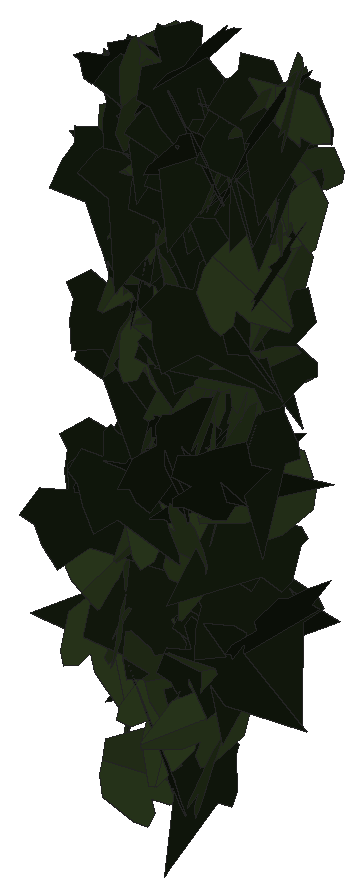
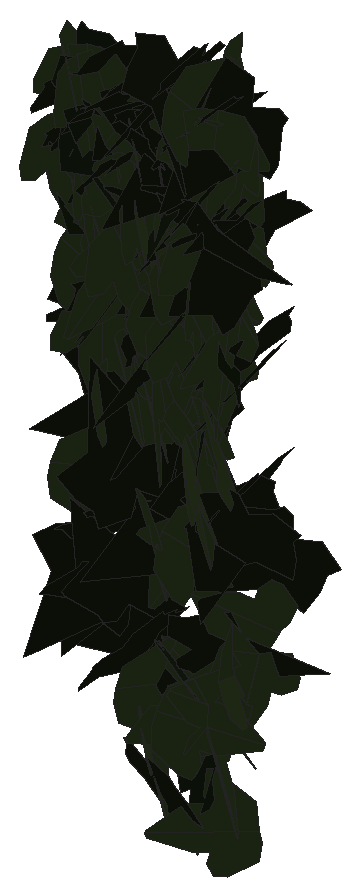
# SketchUp Ruby script. Lengths in inches.
U = 1.inch
M = Sketchup.active_model
def pt(a) = Geom::Point3d.new(a.map { |v| v * U })
def face(e, loops, mat)
  f = e.add_face(loops[0].map { |a| pt(a) })
  loops[1..].each { |l| e.add_face(l.map { |a| pt(a) }).erase! }
  f.material = f.back_material = mat if mat
  f
end
# faces: each face lists its corners as indices into pts; further lists are holes
def faces(e, pts, list, mat = nil) = list.each { |f| face(e, (f[0].is_a?(Array) ? f : [f]).map { |l| l.map { |i| pts[i] } }, mat) }
# xy, xz, yz: faces in a plane at the given z, y or x. An outline is a flat list of corners, or four numbers for a rectangle; further outlines are holes
def ring(l) = l.size == 4 ? [[l[0], l[1]], [l[2], l[1]], [l[2], l[3]], [l[0], l[3]]] : l.each_slice(2).to_a
def flat(e, list, mat, &to3) = list.each { |f| face(e, (f[0].is_a?(Array) ? f : [f]).map { |l| ring(l).map { |u, v| to3.(u, v) } }, mat) }
def xy(e, z, list, mat = nil) = flat(e, list, mat) { |x, y| [x, y, z] }
def xz(e, y, list, mat = nil) = flat(e, list, mat) { |x, z| [x, y, z] }
def yz(e, x, list, mat = nil) = flat(e, list, mat) { |y, z| [x, y, z] }
def lines(e, pts, list) = list.each { |a, b| e.add_line(pt(pts[a]), pt(pts[b])) }
# prism: a flat outline (further loops are holes) pulled along v
def prism(e, loops, v, mat = nil)
  f = face(e, loops, mat); d = Geom::Vector3d.new(v.map { |x| x * U })
  f.pushpull(f.normal.samedirection?(d) ? d.length : -d.length)
end
def box(e, o, s, mat = nil) = prism(e, [[o, [o[0] + s[0], o[1], o[2]], [o[0] + s[0], o[1] + s[1], o[2]], [o[0], o[1] + s[1], o[2]]]], [0, 0, s[2]], mat)
def at(x, y, z, deg = 0) = Geom::Transformation.translation(pt([x, y, z])) * Geom::Transformation.rotation(ORIGIN, Z_AXIS, deg.degrees)
def axes(o, x, y, z) = Geom::Transformation.new([*x, 0, *y, 0, *z, 0, *pt(o).to_a, 1])
def part(name) = M.definitions.add(name)
# library, detail: a bought-in or finely detailed component or shape, given as its bounding box
def library(name, o, s) = part(name).tap { |d| box(d.entities, o, s) }
def detail(e, o, s) = box(e.add_group.entities, o, s)
def put(e, d, t, mat = nil) = e.add_instance(d, t).tap { |i| i.material = mat if mat }
def group(e, t, mat = nil) = e.add_group.tap { |g| g.transformation = t; g.material = mat if mat }.entities
root = M.entities
M.materials.add("efeu1").color = [18, 25, 13]
M.materials.add("efeu2").color = [43, 57, 29]
c1 = part("ivyleaf_9")
p = [[1.54,2.16,1.25],[1.36,2.04,1.19],[-0.21,0.99,0.68],[-0.71,1.11,0.82],[-0.85,0.86,0.67],[-0.8,0.17,0.21],
  [-0.9,-0.01,0.1],[-0.67,-0.16,-0.02],[-0.08,-0.08,-0.05],[-0.03,-0.6,-0.4],[0.65,-0.88,-0.66],[0.83,-0.6,-0.49],
  [1.29,-0.42,-0.43],[1.8125,-0.07,-0.26],[1.21,0.44,0.15]]
faces(c1.entities,p,[[0,1,2,3,4,5,6,7,8,9,10,11,12,13,14]],"efeu1")
c2 = part("ivyleaf_10")
p = [[0,0.5,-0.03],[-0.0625,2.02,-0.43],[-0.19,2.01,-0.46],[-0.54,1.05,-0.29],[-0.52,0.625,-0.18],[-0.83,0.76,-0.28],
  [-1.16,0.64,-0.33],[-1.15,0.33,-0.24],[-0.77,-0.39,0.02],[-0.3,-0.51,0.16],[0.04,-0.48,0.23],[-0.02,2.01,-0.4375],
  [-0.06,2.01,-0.43],[0.04,-0.49,0.23],[0.67,-0.49,0.14],[1.38,0.36,-0.2],[1.375,0.51,-0.24],[0.81,0.65,-0.19],
  [0.62,0.59,-0.15],[0.6,1.09,-0.28],[0.5,1.23,-0.31]]
faces(c2.entities,p,[[0,1,2,3,4,5,6,7,8,9,10],[11,12,0,13,14,15,16,17,18,19,20]],"efeu2")
put(root,c1,axes([30.1875,223.73,218.27],[0.30823,0.1152,0.37646],[0.34662,0.14732,-0.32887],[-0.18669,0.46371,0.01096]))
put(root,c1,axes([30.05,223.875,220.49],[0.05189,-0.28466,-0.40777],[0.01949,0.41083,-0.28432],[0.49692,0.01361,0.05374]))
put(root,c2,axes([29.28,223.65,222.73],[0.01984,-0.0861,-0.49213],[-0.01626,0.49215,-0.08676],[0.49934,0.01944,0.01673]))
put(root,c1,axes([29.74,223.64,218.63],[-0.04067,0.07095,-0.49327],[-0.15542,0.46842,0.08019],[0.47349,0.15985,-0.01604]))
put(root,c1,axes([28.77,223.94,217.97],[0.27322,-0.33997,-0.24448],[-0.06771,0.25221,-0.42639],[0.41324,0.2661,0.09178]))
put(root,c1,axes([28.76,224.29,219.24],[0.07858,-0.48227,0.10603],[0.03475,-0.1017,-0.48831],[0.49256,0.08411,0.01754]))
put(root,c2,axes([30,224.4,215.17],[-0.10002,-0.01335,0.48971],[-0.07704,-0.49317,-0.02918],[0.4838,-0.08129,0.09659]))
put(root,c1,axes([29.83,224.33,222.33],[-0.24105,-0.43748,-0.0226],[0.01521,0.01743,-0.49946],[0.4378,-0.24148,0.0049]))
put(root,c1,axes([29.38,224.24,218.12],[0.19946,-0.19826,0.41341],[0.31844,-0.26446,-0.28047],[0.32987,0.37517,0.02077]))
put(root,c2,axes([29.8,224.47,219.83],[-0.07613,-0.08847,-0.48619],[-0.2503,-0.41725,0.11512],[-0.42609,0.26091,0.01924]))
put(root,c1,axes([29.32,224.45,217.93],[-0.04469,-0.06687,0.49349],[0.07031,-0.49136,-0.06021],[0.49301,0.06401,0.05332]))
put(root,c1,axes([29.86,223.93,222.43],[0.29147,0.04484,-0.40378],[-0.40614,0.04395,-0.2883],[0.00964,0.49604,0.06204]))
put(root,c1,axes([28.29,223.96,217.4],[0.01924,-0.08958,-0.49153],[0.23882,0.43371,-0.0697],[0.43885,-0.2321,0.05947]))
put(root,c2,axes([29.51,224.04,220.53],[-0.38484,0.31191,0.06791],[-0.07388,0.01645,-0.49424],[-0.31055,-0.39043,0.03343]))
put(root,c2,axes([29.62,224.43,219.1],[-0.1673,-0.31373,-0.35155],[-0.17157,-0.30688,0.35551],[-0.43883,0.23958,-0.00497]))
put(root,c2,axes([29.23,224.16,215.33],[-0.2636,-0.10284,0.41224],[0.41013,0.0651,0.27849],[-0.11095,0.48496,0.05004]))
put(root,c1,axes([28.61,224.24,219.85],[0.13988,-0.4487,-0.1706],[-0.039,0.16649,-0.46985],[0.47845,0.14475,0.01158]))
put(root,c1,axes([30.02,224.12,222.24],[0.03969,0.44035,-0.23348],[-0.01765,-0.23283,-0.44213],[-0.49811,0.04334,-0.00294]))
put(root,c1,axes([29.87,224.09,215.95],[0.06492,-0.00021,-0.49577],[0.37049,0.33227,0.04838],[0.32943,-0.37363,0.04329]))
put(root,c2,axes([30.46,223.94,220.87],[0.12331,0.35,0.3351],[0.09963,0.32008,-0.37097],[-0.4742,0.15826,0.0092]))
put(root,c1,axes([28.61,224.42,221.43],[-0.10626,-0.48093,-0.08611],[0.00554,0.08694,-0.49235],[0.48855,-0.10559,-0.01315]))
put(root,c2,axes([29.96,224.29,219.05],[0.23522,-0.43747,-0.05737],[-0.03723,0.0451,-0.49657],[0.43964,0.23788,-0.01135]))
put(root,c1,axes([29.8125,224.45,221.89],[-0.04801,-0.49268,-0.07041],[0.01432,0.06934,-0.49496],[0.49748,-0.04955,0.00746]))
put(root,c1,axes([29.07,224.57,222.47],[-0.09606,-0.47998,0.10192],[0.0028,-0.10439,-0.48897],[0.49068,-0.09337,0.02274]))
put(root,c1,axes([29.36,224.27,214.17],[0.16983,-0.32992,0.33513],[-0.1158,0.316,0.36977],[-0.45579,-0.20322,0.03092]))
put(root,c2,axes([29.8,224.1,217.06],[0.11381,-0.1009,-0.4763],[-0.36795,0.30251,-0.152],[0.31884,0.38511,-0.0054]))
put(root,c1,axes([28.9,224.59,221.3],[-0.15182,-0.4695,0.08071],[-0.01491,-0.07999,-0.49333],[0.47616,-0.15221,0.01029]))
put(root,c1,axes([30.49,224.4,218.87],[-0.31705,-0.08095,-0.37806],[0.36567,0.096,-0.32721],[0.12557,-0.48397,-0.00167]))
put(root,c2,axes([28.54,224.23,215.86],[0.2873,0.39943,0.08896],[0.04726,0.07558,-0.49199],[-0.40648,0.29111,0.00567]))
put(root,c2,axes([29.93,224.31,214.68],[0.20561,-0.44822,-0.08263],[-0.04335,0.071,-0.49303],[0.4537,0.20991,-0.00967]))
put(root,c1,axes([29.16,224.45,215.97],[-0.32167,-0.01003,0.38266],[-0.38267,-0.00433,-0.32179],[0.00977,-0.49988,-0.0049]))
put(root,c2,axes([29.6,224.44,219.01],[-0.31988,-0.21954,0.3154],[-0.2488,-0.19443,-0.38768],[0.29287,-0.40497,0.01515]))
put(root,c1,axes([28.78,224.52,220.21],[0.19828,-0.4454,0.11092],[0.03823,-0.10438,-0.48749],[0.45741,0.20179,-0.00734]))
put(root,c1,axes([30.43,224.54,222.28],[-0.0464,-0.49705,-0.028],[-0.00153,0.02826,-0.4992],[0.49784,-0.04624,-0.00414]))
put(root,c2,axes([29.15,224.35,218.8],[0.39495,-0.28137,-0.12183],[-0.09512,0.07644,-0.48488],[0.29149,0.40619,0.00685]))
put(root,c2,axes([28.98,224.54,220.58],[0.16357,0.32776,-0.34032],[-0.18287,-0.28816,-0.36541],[-0.43567,0.24401,0.0256]))
put(root,c2,axes([30.03,224.37,221.95],[0.22572,-0.4388,-0.08062],[-0.04065,0.06975,-0.49344],[0.44429,0.22932,-0.00419]))
put(root,c2,axes([28.47,224.52,220.23],[0.18963,-0.13955,-0.4411],[0.35215,-0.26564,0.23543],[-0.30006,-0.39995,-0.00246]))
put(root,c2,axes([28.91,224.24,219.64],[0.07968,-0.44012,-0.22349],[0.00451,0.22702,-0.44547],[0.49359,0.06898,0.04014]))
put(root,c2,axes([30.54,224.35,219.59],[-0.33784,-0.36837,-0.01319],[0.00837,0.01021,-0.49983],[0.36851,-0.33794,-0.00073]))
put(root,c1,axes([29.77,224.37,219.52],[-0.20294,-0.40635,0.20905],[0.12789,0.16909,0.45283],[-0.4387,0.23726,0.03531]))
put(root,c1,axes([28.9,224.14,217.875],[0.27649,0.40731,-0.08747],[-0.04935,-0.07222,-0.49229],[-0.41366,0.28086,0.00027]))
put(root,c1,axes([29.4375,224.11,222.98],[0.29733,-0.13893,-0.37722],[-0.17794,0.37524,-0.27845],[0.36046,0.29983,0.1737]))
put(root,c2,axes([29.13,224.67,222.81],[-0.00769,-0.35915,0.34778],[0.02542,-0.34765,-0.35846],[0.49929,0.01217,0.02361]))
put(root,c1,axes([30.7,224.66,219.77],[-0.35779,-0.08307,0.33925],[-0.30073,-0.17371,-0.3597],[0.17762,-0.46144,0.07434]))
put(root,c2,axes([29.17,224.27,219.6],[0.16895,0.45543,0.11848],[0.04351,0.11023,-0.48575],[-0.46857,0.17445,-0.00238]))
put(root,c2,axes([29.32,224.44,215.08],[0.38699,0.3021,-0.09474],[-0.07432,-0.05877,-0.49094],[-0.30776,0.39406,-0.00058]))
put(root,c2,axes([30.33,224.52,218.8125],[0.12888,-0.47641,0.08012],[0.02461,-0.07634,-0.49352],[0.48248,0.13116,0.00377]))
put(root,c1,axes([29.19,224.59,221.3],[0.11792,-0.48582,0.00842],[0.00252,-0.00805,-0.49993],[0.48589,0.11795,0.00055]))
put(root,c1,axes([30.88,224.39,221.11],[-0.33212,0.36284,-0.08968],[0.06125,-0.06551,-0.49189],[-0.36871,-0.33772,-0.00093]))
put(root,c2,axes([28.49,224.73,215.96],[0.12848,-0.12607,0.46647],[0.29574,-0.36121,-0.17908],[0.38214,0.32192,-0.01825]))
put(root,c2,axes([29.15,224.73,217.41],[-0.03937,-0.31933,0.38272],[-0.0593,-0.37819,-0.32165],[0.49491,-0.07072,-0.00809]))
put(root,c1,axes([30.66,224.58,222.75],[-0.25851,0.25501,-0.34372],[0.20541,-0.27836,-0.361],[-0.37547,-0.32785,0.03915]))
put(root,c2,axes([28.72,224.58,221.25],[0.42305,-0.1473,0.22211],[0.20666,-0.0818,-0.44788],[0.16828,0.47076,-0.00832]))
put(root,c1,axes([30.3,224.72,222.38],[-0.03734,-0.49582,0.0526],[0.0055,-0.05316,-0.49714],[0.49857,-0.03655,0.00943]))
put(root,c2,axes([29.4,224.57,218.93],[0.34869,-0.07996,0.34931],[0.34267,-0.06817,-0.35767],[0.10482,0.48883,0.00725]))
put(root,c2,axes([28.82,224.4,222.03],[-0.42019,-0.09996,-0.25189],[0.25346,0.01953,-0.43056],[0.09592,-0.48952,0.03426]))
put(root,c1,axes([28.96,224.11,219.72],[-0.02814,0.12586,0.48308],[-0.03925,0.48179,-0.12781],[-0.49766,-0.04512,-0.01724]))
put(root,c1,axes([30.45,224.79,222.21],[-0.19949,-0.44781,0.09833],[-0.00418,-0.10546,-0.48873],[0.45846,-0.19582,0.03834]))
put(root,c1,axes([30.27,224.83,217.36],[-0.37185,-0.27641,0.18796],[-0.07734,-0.20238,-0.45062],[0.32519,-0.3642,0.10776]))
put(root,c2,axes([28.65,224.41,222.38],[-0.46189,0.19111,-0.01173],[0.00851,-0.0101,-0.49983],[-0.19128,-0.46193,0.00608]))
put(root,c1,axes([29.58,224.26,222.95],[-0.04809,0.49724,0.02099],[-0.00324,0.02077,-0.49956],[-0.49767,-0.04818,0.00123]))
put(root,c2,axes([28.45,224.19,216.39],[0.18399,0.21379,-0.41285],[0.2775,0.30574,0.28199],[0.37302,-0.33289,-0.00615]))
put(root,c1,axes([30.53,224.75,222.74],[-0.12511,-0.48402,0.00848],[-0.00193,-0.00826,-0.49993],[0.48409,-0.12513,0.0002]))
put(root,c1,axes([30.16,224.54,220.12],[0.29469,-0.39669,-0.07609],[-0.03476,0.06894,-0.494],[0.40243,0.29645,0.01306]))
put(root,c2,axes([29.46,224.55,221.17],[0.11766,-0.48577,-0.01339],[0.00267,0.01442,-0.49978],[0.48595,0.11754,0.00599]))
put(root,c2,axes([29,224.52,222.43],[0.48556,0.09732,0.06897],[0.06686,0.01738,-0.4952],[-0.09879,0.49013,0.00386]))
put(root,c1,axes([29.64,224.66,214.4375],[-0.43821,-0.01485,-0.24032],[0.2404,0.00085,-0.43841],[0.01343,-0.49978,0.00639]))
put(root,c1,axes([28.7,224.64,221.99],[0.16868,-0.46834,-0.04695],[-0.00793,0.04704,-0.49772],[0.47062,0.16866,0.00844]))
put(root,c1,axes([28.63,224.25,222.72],[0.433,0.24663,0.04106],[0.03279,0.02539,-0.49828],[-0.24787,0.4342,0.00581]))
put(root,c2,axes([30.61,224.57,222.7],[-0.47651,-0.14983,0.02208],[0.0209,-0.13726,-0.48034],[0.15,-0.45685,0.13707]))
put(root,c2,axes([30.53,224.84,217.91],[-0.10569,-0.05565,0.48552],[-0.18342,-0.45591,-0.09219],[0.45297,-0.1976,0.07595]))
put(root,c1,axes([30.01,224.61,221.75],[0.02863,-0.46877,-0.17156],[-0.01021,0.17126,-0.46964],[0.49908,0.0304,0.00023]))
put(root,c2,axes([29.06,224.61,218.43],[0.18863,-0.46188,0.03291],[0.00319,-0.03424,-0.49882],[0.46304,0.18839,-0.00997]))
put(root,c1,axes([28.42,224.52,217.89],[-0.14631,-0.21065,-0.42921],[0.30723,0.3025,-0.25319],[0.36634,-0.33782,0.04091]))
put(root,c1,axes([29.42,224.55,215.79],[-0.44323,0.23113,0.01139],[-0.01099,0.00356,-0.49987],[-0.23115,-0.44336,0.00192]))
put(root,c1,axes([29.39,224.28,219.73],[0.23643,-0.16463,-0.40865],[-0.1363,0.41369,-0.24552],[0.41895,0.2275,0.15074]))
put(root,c1,axes([29.01,224.73,220.38],[0.15164,-0.47598,0.02125],[-0.00528,-0.02397,-0.4994],[0.47642,0.15124,-0.0123]))
put(root,c2,axes([29.86,224.51,221.78],[-0.4396,0.22169,0.0872],[-0.12104,-0.05021,-0.48252],[-0.20518,-0.44535,0.09781]))
put(root,c1,axes([30.26,224.58,216.56],[-0.05408,-0.3896,-0.30869],[0.08894,0.29792,-0.39158],[0.48905,-0.09726,0.03707]))
put(root,c2,axes([30.2,224.39,219.17],[0.18227,-0.25432,-0.39],[-0.23304,0.31274,-0.31286],[0.40307,0.29582,-0.00453]))
put(root,c2,axes([29.17,224.37,217.35],[0.1718,0.3913,0.25955],[0.10645,0.23672,-0.42735],[-0.45733,0.2021,-0.00197]))
put(root,c2,axes([28.8,224.43,221.2],[-0.30316,-0.29068,-0.2713],[0.21412,0.16812,-0.41939],[0.33504,-0.37046,0.02254]))
put(root,c2,axes([28.99,224.56,220.49],[0.08937,-0.48461,-0.08466],[0.04489,0.09372,-0.48908],[0.4899,0.07982,0.06026]))
put(root,c2,axes([30.51,224.88,220.625],[-0.04312,-0.34729,0.35711],[0.12884,-0.35403,-0.32873],[0.48119,0.06367,0.12002]))
put(root,c1,axes([29.63,224.79,221.52],[-0.4378,-0.23106,-0.07035],[0.07015,0.0177,-0.49474],[0.23111,-0.44306,0.01692]))
put(root,c1,axes([30.11,224.73,222.2],[-0.37042,-0.14873,-0.30111],[0.29164,0.07985,-0.39821],[0.16654,-0.47064,0.02759]))
put(root,c1,axes([29.12,224.31,222.16],[0.44262,0.19608,0.12506],[0.10557,0.07017,-0.48366],[-0.20723,0.45456,0.02071]))
put(root,c2,axes([29.05,224.79,220.9],[-0.19311,-0.3888,0.24808],[-0.08446,-0.23459,-0.4334],[0.4534,-0.20929,0.02493]))
put(root,c2,axes([29.1,224.78,220.13],[-0.21763,-0.39389,0.21791],[-0.02769,-0.22987,-0.44316],[0.4493,-0.20496,0.07824]))
put(root,c2,axes([28.71,224.55,218.33],[0.36564,-0.33529,0.06238],[-0.03642,0.05255,0.4959],[-0.33909,-0.36718,0.014]))
put(root,c2,axes([30.8,224.61,221.76],[0.33801,0.01111,-0.36828],[-0.36645,0.06207,-0.33446],[0.03828,0.49601,0.0501]))
put(root,c2,axes([28.625,224.43,213.93],[0.08217,-0.01615,0.49294],[0.40103,0.29309,-0.05725],[-0.2871,0.40477,0.06112]))
put(root,c2,axes([30.46,224.5,221.51],[-0.33949,0.18139,0.31913],[-0.3245,0.0549,-0.37641],[-0.17159,-0.46269,0.08045]))
put(root,c2,axes([28.88,224.64,221.05],[-0.31063,-0.39052,0.03162],[-0.02051,-0.02408,-0.499],[0.39126,-0.31131,-0.00106]))
put(root,c1,axes([29.79,224.92,215.98],[-0.03953,-0.4893,0.09497],[0.01224,-0.09619,-0.49051],[0.49828,-0.03645,0.01958]))
put(root,c2,axes([29.3125,224.95,220.4375],[-0.17256,-0.28896,0.36976],[0.03591,-0.40095,-0.29657],[0.4679,-0.07579,0.15913]))
put(root,c1,axes([30.44,224.51,222],[-0.16051,0.46988,-0.05875],[-0.03564,-0.07384,-0.49323],[-0.47219,-0.15415,0.05719]))
put(root,c2,axes([29.01,224.66,218.25],[0.163,-0.46836,-0.06382],[-0.02811,0.05778,-0.49585],[0.47185,0.16523,-0.00749]))
put(root,c2,axes([30.11,224.73,221.11],[-0.4668,-0.12528,-0.12809],[0.16484,-0.16022,-0.44402],[0.07021,-0.45676,0.19088]))
put(root,c2,axes([28.81,224.62,222.53],[-0.47704,-0.1496,0.00742],[-0.00708,-0.00221,-0.49994],[0.14962,-0.47709,-0.00001]))
put(root,c1,axes([29.31,224.66,221.55],[0.37093,-0.32626,-0.07725],[-0.0635,0.04476,-0.49393],[0.32921,0.37624,-0.00823]))
put(root,c2,axes([29.66,224.76,221.375],[0.02551,-0.49578,0.05962],[0.00963,-0.0592,-0.49639],[0.49926,0.02647,0.00653]))
put(root,c1,axes([30.61,224.27,216.42],[0.19835,0.38003,0.25736],[0.1073,0.2342,-0.42853],[-0.44625,0.22523,0.01135]))
put(root,c2,axes([30.74,224.31,221.63],[-0.01014,0.09623,-0.49055],[-0.08725,0.48278,0.09651],[0.49222,0.08756,0.007]))
put(root,c2,axes([30.14,224.71,222.03],[0.38952,0.02317,0.31263],[0.31213,0.01758,-0.39021],[-0.02907,0.49915,-0.00077]))
put(root,c2,axes([30.6875,224.75,222.89],[0.27408,-0.41793,0.01449],[0.04161,0.01002,-0.49817],[0.41611,0.27428,0.04027]))
put(root,c2,axes([30.4,224.69,221.54],[0.06376,-0.4916,-0.06527],[0.0277,0.06924,-0.49441],[0.49514,0.05943,0.03607]))
put(root,c2,axes([30.42,224.76,221.4],[0.2885,-0.40825,-0.01001],[-0.0148,0.00179,-0.49978],[0.4081,0.28867,-0.01105]))
put(root,c2,axes([30.73,224.75,221.91],[-0.27006,-0.41814,0.04714],[-0.0144,-0.0468,-0.4976],[0.42055,-0.27012,0.01323]))
put(root,c2,axes([29.62,224.76,221.35],[0.19848,-0.45862,-0.01647],[-0.01095,0.01321,-0.49971],[0.45879,0.19872,-0.0048]))
put(root,c1,axes([29.99,224.61,216.37],[-0.31229,-0.01189,0.3903],[0.38885,-0.05508,0.30945],[0.03564,0.49681,0.04365]))
put(root,c2,axes([29.67,224.72,217.66],[0.31324,-0.36453,-0.13783],[-0.09082,0.10368,-0.48063],[0.37899,0.32614,-0.00126]))
put(root,c1,axes([29.35,224.34,217.46],[0.25298,0.27648,0.331],[0.21876,0.24845,-0.37472],[-0.37168,0.33441,0.00474]))
put(root,c2,axes([29.81,224.85,220.91],[-0.26395,-0.40372,0.13167],[-0.02022,-0.14291,-0.47872],[0.42417,-0.25804,0.05911]))
put(root,c1,axes([29.78,224.74,217.92],[0.31705,0.35367,0.15619],[-0.1091,-0.11195,0.47494],[0.37092,-0.33523,0.00618]))
put(root,c2,axes([28.59,224.81,215.06],[0.28759,-0.409,0.0027],[0.0017,-0.0021,-0.49999],[0.40901,0.28759,0.00018]))
put(root,c2,axes([30.49,224.76,222.68],[-0.04018,-0.49769,-0.02637],[-0.00414,0.02678,-0.49926],[0.49837,-0.0399,-0.00628]))
put(root,c2,axes([29.64,224.57,219.03],[0.2317,-0.30263,-0.32362],[-0.13448,0.29993,-0.37677],[0.42217,0.26163,0.05759]))
put(root,c2,axes([29.8125,224.74,221.71],[-0.435,-0.22807,0.09357],[-0.08637,-0.03674,-0.49111],[0.23089,-0.44343,-0.00743]))
put(root,c2,axes([30.1,224.56,220.5],[-0.1901,-0.33646,-0.31727],[0.20475,0.24635,-0.38392],[0.41466,-0.27588,0.04412]))
put(root,c2,axes([28.69,224.48,215.36],[0.01264,-0.30445,0.39642],[-0.02857,0.39546,0.30462],[-0.49902,-0.03035,-0.0074]))
put(root,c2,axes([28.57,224.72,220.09],[-0.03834,0.49813,-0.01984],[-0.04101,-0.02299,-0.49778],[-0.49684,-0.03655,0.04262]))
put(root,c2,axes([28.9,225.08,215.47],[-0.07647,-0.17921,0.46047],[-0.19472,-0.41732,-0.19476],[0.45413,-0.20912,-0.00597]))
put(root,c1,axes([29.02,224.71,221.26],[-0.26668,0.16993,0.38731],[-0.34247,0.18192,-0.31562],[-0.24819,-0.43362,0.01937]))
put(root,c1,axes([28.47,224.65,221.0625],[0.4769,-0.02872,0.14745],[0.14666,-0.01719,-0.4777],[0.03251,0.49888,-0.00797]))
